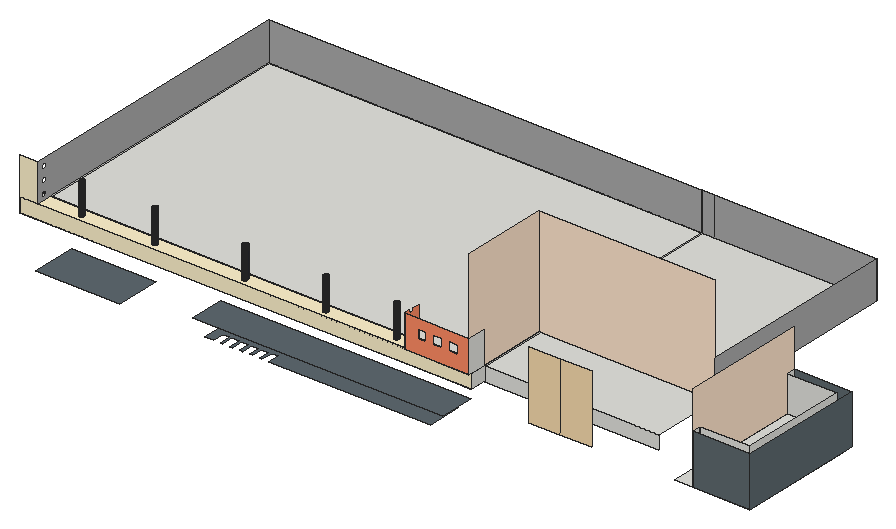
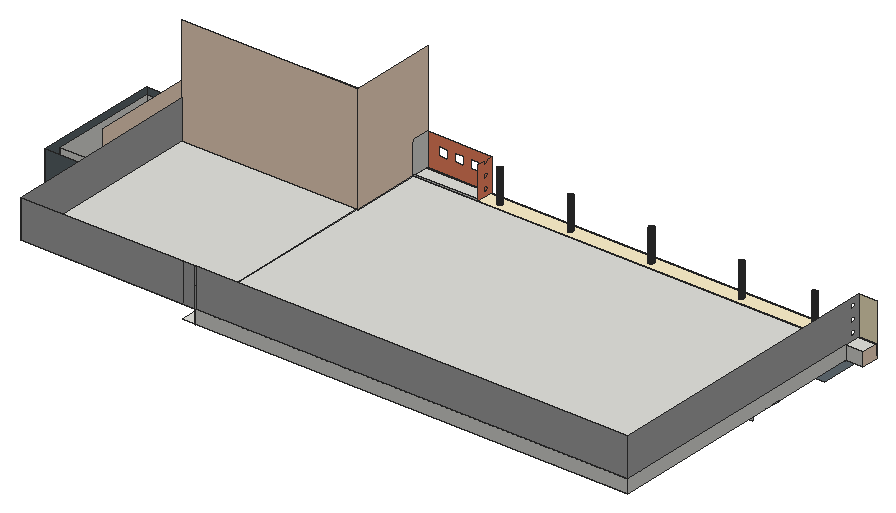
# SketchUp Ruby script. Lengths in inches.
U = 1.inch
M = Sketchup.active_model
def pt(a) = Geom::Point3d.new(a.map { |v| v * U })
def face(e, loops, mat)
  f = e.add_face(loops[0].map { |a| pt(a) })
  loops[1..].each { |l| e.add_face(l.map { |a| pt(a) }).erase! }
  f.material = f.back_material = mat if mat
  f
end
# faces: each face lists its corners as indices into pts; further lists are holes
def faces(e, pts, list, mat = nil) = list.each { |f| face(e, (f[0].is_a?(Array) ? f : [f]).map { |l| l.map { |i| pts[i] } }, mat) }
# xy, xz, yz: faces in a plane at the given z, y or x. An outline is a flat list of corners, or four numbers for a rectangle; further outlines are holes
def ring(l) = l.size == 4 ? [[l[0], l[1]], [l[2], l[1]], [l[2], l[3]], [l[0], l[3]]] : l.each_slice(2).to_a
def flat(e, list, mat, &to3) = list.each { |f| face(e, (f[0].is_a?(Array) ? f : [f]).map { |l| ring(l).map { |u, v| to3.(u, v) } }, mat) }
def xy(e, z, list, mat = nil) = flat(e, list, mat) { |x, y| [x, y, z] }
def xz(e, y, list, mat = nil) = flat(e, list, mat) { |x, z| [x, y, z] }
def yz(e, x, list, mat = nil) = flat(e, list, mat) { |y, z| [x, y, z] }
def lines(e, pts, list) = list.each { |a, b| e.add_line(pt(pts[a]), pt(pts[b])) }
# prism: a flat outline (further loops are holes) pulled along v
def prism(e, loops, v, mat = nil)
  f = face(e, loops, mat); d = Geom::Vector3d.new(v.map { |x| x * U })
  f.pushpull(f.normal.samedirection?(d) ? d.length : -d.length)
end
def box(e, o, s, mat = nil) = prism(e, [[o, [o[0] + s[0], o[1], o[2]], [o[0] + s[0], o[1] + s[1], o[2]], [o[0], o[1] + s[1], o[2]]]], [0, 0, s[2]], mat)
def at(x, y, z, deg = 0) = Geom::Transformation.translation(pt([x, y, z])) * Geom::Transformation.rotation(ORIGIN, Z_AXIS, deg.degrees)
def axes(o, x, y, z) = Geom::Transformation.new([*x, 0, *y, 0, *z, 0, *pt(o).to_a, 1])
def part(name) = M.definitions.add(name)
# library, detail: a bought-in or finely detailed component or shape, given as its bounding box
def library(name, o, s) = part(name).tap { |d| box(d.entities, o, s) }
def detail(e, o, s) = box(e.add_group.entities, o, s)
def put(e, d, t, mat = nil) = e.add_instance(d, t).tap { |i| i.material = mat if mat }
def group(e, t, mat = nil) = e.add_group.tap { |g| g.transformation = t; g.material = mat if mat }.entities
root = M.entities
M.materials.add("[Color B03]").color = [255, 140, 101]
M.materials.add("[Color C01]1").color = [255, 229, 204]
M.materials.add("[Color D01]").color = [255, 242, 204]
M.materials.add("[Color M03]").color = [170, 170, 170]
M.materials.add("[Formica Beige]1").color = [247, 219, 174]
M.materials.add("[Formica Laminate Dark]").color = [50, 53, 60]
M.materials.add("[Formica Speckled Grey]").color = [94, 105, 111]
xy(root,885.007,[[1665.331,219.809,1713.027,557.621],[1713.027,528.448,1866.152,557.621]])
xy(root,885.007,[[[1713.027,219.809,1713.027,240.489,1736.964,240.489,1736.964,274.614,1713.027,274.614,1713.027,528.448,1866.152,528.448,1866.152,219.809],[1750.402,240.489,1774.339,274.614],[1790.964,240.489,1814.902,274.614],[1823.339,240.489,1847.277,274.614]]],"[Formica Speckled Grey]")
xy(root,892.389,[[531.184,73.923,531.184,166.105,1131.08,166.105,1131.08,73.923,701.834,73.923,701.834,104.16,683.146,104.16,683.146,73.923,676.459,73.923,676.459,104.16,657.771,104.16,657.771,73.923,650.271,73.923,650.271,104.16,631.584,104.16,631.584,73.923,623.459,73.923,623.459,104.16,604.771,104.16,604.771,73.923,597.959,73.923,597.959,104.16,579.271,104.16,579.271,73.923,572.521,73.923,572.521,104.16,553.834,104.16,553.834,73.923]],"[Formica Speckled Grey]")
xy(root,911.081,[[100.986,47.542,326.111,166.105]],"[Formica Speckled Grey]")
xy(root,922.568,[[1713.027,243.888,1844.714,533.576]])
xy(root,925.697,[[497.875,73.923,1164.389,166.105]],"[Formica Speckled Grey]")
xy(root,980.3125,[[1198.268,166.042,1198.268,166.105,451.357,166.105,451.357,166.083,497.875,166.08],[1201.787,166.042,1232.713,890.389],[451.357,166.083,451.357,166.105,47.696,166.105],[1198.268,351.292,1201.787,388.542],[47.696,388.542,1201.412,388.542,1201.412,890.389,1198.268,890.389,1198.268,436.378,47.696,436.378]])
xy(root,980.9375,[[0,122.542,0,166.105,47.696,166.105,412.335,166.085,412.335,122.542],[412.335,122.542,412.335,166.085,451.311,166.083,451.311,122.542],[451.311,122.542,451.311,166.083,497.875,166.08,1159.05,166.044,1159.05,122.542],[1159.05,122.542,1159.05,166.044,1198.268,166.042,1198.268,122.542],[1198.268,122.542,1201.787,890.389],
  [1198.268,166.042,1159.05,166.044,1159.05,436.378,1198.268,436.378],[1159.05,166.044,497.875,166.08,451.311,166.083,451.311,436.378,1159.05,436.378],[451.311,166.083,412.335,166.085,412.335,436.378,451.311,436.378],[412.335,166.085,47.696,166.105,47.696,436.378,412.335,436.378],[47.696,436.378,412.335,890.389],
  [412.335,436.378,451.311,890.389],[451.311,436.378,1159.05,890.389],[1159.05,436.378,1198.268,890.389]])
xy(root,1016.9375,[[1025.893,119.173,1198.268,122.542],[0,122.542,47.696,166.105],[1198.268,122.542,1201.787,122.542,1201.787,890.389,47.696,890.389,47.696,166.105,1198.268,166.042],[1025.893,122.542,1198.268,166.042],[147.908,137.16,146.226,137.382,144.658,138.031,143.312,139.064,142.279,140.41,141.63,141.978,141.408,143.66,141.63,145.343,142.279,146.91,143.312,148.257,144.658,149.289,146.226,149.939,147.908,150.16,149.591,149.939,151.158,149.289,152.504,148.257,153.537,146.91,154.187,145.343,154.408,143.66,154.187,141.978,153.537,140.41,152.504,139.064,151.158,138.031,149.591,137.382],
  [341.783,137.16,340.101,137.382,338.533,138.031,337.187,139.064,336.154,140.41,335.505,141.978,335.283,143.66,335.505,145.343,336.154,146.91,337.187,148.257,338.533,149.289,340.101,149.939,341.783,150.16,343.466,149.939,345.033,149.289,346.379,148.257,347.412,146.91,348.062,145.343,348.283,143.66,348.062,141.978,347.412,140.41,346.379,139.064,345.033,138.031,343.466,137.382],[582.033,137.16,580.351,137.382,578.783,138.031,577.437,139.064,576.404,140.41,575.755,141.978,575.533,143.66,575.755,145.343,576.404,146.91,577.437,148.257,578.783,149.289,580.351,149.939,582.033,150.16,583.716,149.939,585.283,149.289,586.629,148.257,587.662,146.91,588.312,145.343,588.533,143.66,588.312,141.978,587.662,140.41,586.629,139.064,585.283,138.031,583.716,137.382],[797.721,137.16,796.038,137.382,794.471,138.031,793.125,139.064,792.092,140.41,791.442,141.978,791.221,143.66,791.442,145.343,792.092,146.91,793.125,148.257,794.471,149.289,796.038,149.939,797.721,150.16,799.403,149.939,800.971,149.289,802.317,148.257,803.35,146.91,803.999,145.343,804.221,143.66,803.999,141.978,803.35,140.41,802.317,139.064,800.971,138.031,799.403,137.382],[984.137,138.709,982.455,138.93,980.887,139.58,979.541,140.613,978.508,141.959,977.859,143.527,977.637,145.209,977.859,146.891,978.508,148.459,979.541,149.805,980.887,150.838,982.455,151.487,984.137,151.709,985.819,151.487,987.387,150.838,988.733,149.805,989.766,148.459,990.416,146.891,990.637,145.209,990.416,143.527,989.766,141.959,988.733,140.613,987.387,139.58,985.819,138.93],[1201.787,166.042,1665.331,351.292],
  [1201.787,351.292,1665.331,890.389]])
xy(root,1016.9375,[[[47.696,122.542,1025.893,122.542,1025.893,166.042,1198.268,166.042,47.696,166.105],[984.137,138.709,982.455,138.93,980.887,139.58,979.541,140.613,978.508,141.959,977.859,143.527,977.637,145.209,977.859,146.891,978.508,148.459,979.541,149.805,980.887,150.838,982.455,151.487,984.137,151.709,985.819,151.487,987.387,150.838,988.733,149.805,989.766,148.459,990.416,146.891,990.637,145.209,990.416,143.527,989.766,141.959,988.733,140.613,987.387,139.58,985.819,138.93],[341.783,137.16,340.101,137.382,338.533,138.031,337.187,139.064,336.154,140.41,335.505,141.978,335.283,143.66,335.505,145.343,336.154,146.91,337.187,148.257,338.533,149.289,340.101,149.939,341.783,150.16,343.466,149.939,345.033,149.289,346.379,148.257,347.412,146.91,348.062,145.343,348.283,143.66,348.062,141.978,347.412,140.41,346.379,139.064,345.033,138.031,343.466,137.382],[797.721,137.16,796.038,137.382,794.471,138.031,793.125,139.064,792.092,140.41,791.442,141.978,791.221,143.66,791.442,145.343,792.092,146.91,793.125,148.257,794.471,149.289,796.038,149.939,797.721,150.16,799.403,149.939,800.971,149.289,802.317,148.257,803.35,146.91,803.999,145.343,804.221,143.66,803.999,141.978,803.35,140.41,802.317,139.064,800.971,138.031,799.403,137.382],[582.033,137.16,580.351,137.382,578.783,138.031,577.437,139.064,576.404,140.41,575.755,141.978,575.533,143.66,575.755,145.343,576.404,146.91,577.437,148.257,578.783,149.289,580.351,149.939,582.033,150.16,583.716,149.939,585.283,149.289,586.629,148.257,587.662,146.91,588.312,145.343,588.533,143.66,588.312,141.978,587.662,140.41,586.629,139.064,585.283,138.031,583.716,137.382],[147.908,137.16,146.226,137.382,144.658,138.031,143.312,139.064,142.279,140.41,141.63,141.978,141.408,143.66,141.63,145.343,142.279,146.91,143.312,148.257,144.658,149.289,146.226,149.939,147.908,150.16,149.591,149.939,151.158,149.289,152.504,148.257,153.537,146.91,154.187,145.343,154.408,143.66,154.187,141.978,153.537,140.41,152.504,139.064,151.158,138.031,149.591,137.382]]],"[Color D01]")
xz(root,119.173,[[[1025.893,1016.9375,1198.268,1102.645],[1060.122,1053.817,1083.872,1077.567],[1102.122,1053.817,1125.872,1077.567],[1144.684,1053.817,1168.434,1077.567]]],"[Color B03]")
xz(root,119.173,[[1358.015,957.692,1440.68,1139.823],[1440.68,957.692,1523.345,1139.823]],"[Formica Beige]1")
xz(root,122.542,[[0,980.9375,1201.787,1016.9375],[0,1016.9375,47.696,1119.0625]],"[Color D01]")
xz(root,166.042,[[1201.787,980.3125,1665.331,1016.9375],[1025.893,1016.9375,1198.268,1021.906]])
xz(root,166.105,[[0,980.9375,47.696,1016.9375]])
xz(root,219.809,[[1713.027,885.007,1866.152,1017.818]],"[Formica Speckled Grey]")
xz(root,243.888,[[1713.027,922.568,1844.714,1017.818]])
xz(root,351.292,[[1198.268,980.3125,1198.268,1305.375,1665.331,1305.375,1665.331,1016.9375,1201.787,1016.9375,1201.787,980.3125]],"[Color C01]1")
xz(root,388.542,[[116.162,908.992,307.287,929.242]])
xz(root,436.378,[[47.696,980.3125,412.335,980.9375],[412.335,980.3125,451.311,980.9375],[451.311,980.3125,1159.05,980.9375],[1159.05,980.3125,1198.268,980.9375]])
xz(root,533.576,[[1713.027,922.568,1844.714,1017.818]])
xz(root,557.621,[[1713.027,885.007,1866.152,1017.818]],"[Formica Speckled Grey]")
xz(root,890.389,[[47.696,980.9375,1201.787,1016.9375]])
xz(root,890.389,[[47.696,1016.9375,1198.268,1119.0625],[1198.268,1016.9375,1201.787,1119.0625],[1201.787,1016.9375,1232.713,1119.0625],[1232.713,1016.9375,1665.331,1119.0625]],"[Color M03]")
yz(root,0,[[122.542,980.9375,166.105,1016.9375]],"[Color C01]1")
yz(root,47.696,[[388.542,980.3125,436.378,980.9375],[166.105,980.9375,890.389,1016.9375]])
yz(root,47.696,[[[122.542,1016.9375,890.389,1119.0625],[141.311,1027.741,139.531,1027.975,137.873,1028.662,136.449,1029.754,135.357,1031.178,134.67,1032.836,134.436,1034.616,134.67,1036.395,135.357,1038.053,136.449,1039.477,137.873,1040.57,139.531,1041.256,141.311,1041.491,143.09,1041.256,144.748,1040.57,146.172,1039.477,147.265,1038.053,147.952,1036.395,148.186,1034.616,147.952,1032.836,147.265,1031.178,146.172,1029.754,144.748,1028.662,143.09,1027.975],[141.311,1060.553,139.531,1060.787,137.873,1061.474,136.449,1062.567,135.357,1063.991,134.67,1065.649,134.436,1067.428,134.67,1069.208,135.357,1070.866,136.449,1072.29,137.873,1073.382,139.531,1074.069,141.311,1074.303,143.09,1074.069,144.748,1073.382,146.172,1072.29,147.265,1070.866,147.952,1069.208,148.186,1067.428,147.952,1065.649,147.265,1063.991,146.172,1062.567,144.748,1061.474,143.09,1060.787],[141.311,1093.991,139.531,1094.225,137.873,1094.912,136.449,1096.004,135.357,1097.428,134.67,1099.086,134.436,1100.866,134.67,1102.645,135.357,1104.303,136.449,1105.727,137.873,1106.82,139.531,1107.506,141.311,1107.741,143.09,1107.506,144.748,1106.82,146.172,1105.727,147.265,1104.303,147.952,1102.645,148.186,1100.866,147.952,1099.086,147.265,1097.428,146.172,1096.004,144.748,1094.912,143.09,1094.225]]],"[Color M03]")
yz(root,1025.893,[[[119.173,1016.9375,119.173,1102.645,134.67,1102.645,134.669,1102.638,134.436,1100.866,134.669,1099.094,134.67,1099.086,135.357,1097.428,136.449,1096.004,137.873,1094.912,139.531,1094.225,141.311,1093.991,143.09,1094.225,144.748,1094.912,146.172,1096.004,147.265,1097.428,147.952,1099.086,147.952,1099.094,148.186,1100.866,147.952,1102.638,147.952,1102.645,166.042,1102.645,166.042,1016.9375],[141.311,1060.553,143.09,1060.787,144.748,1061.474,146.172,1062.567,147.265,1063.991,147.952,1065.649,148.186,1067.428,147.952,1069.208,147.265,1070.866,146.172,1072.29,144.748,1073.382,143.09,1074.069,141.311,1074.303,139.531,1074.069,137.873,1073.382,136.449,1072.29,135.357,1070.866,134.67,1069.208,134.436,1067.428,134.67,1065.649,135.357,1063.991,136.449,1062.567,137.873,1061.474,139.531,1060.787],[141.311,1027.741,143.09,1027.975,144.748,1028.662,146.172,1029.754,147.265,1031.178,147.952,1032.836,148.186,1034.616,147.952,1036.395,147.265,1038.053,146.172,1039.477,144.748,1040.57,143.09,1041.256,141.311,1041.491,139.531,1041.256,137.873,1040.57,136.449,1039.477,135.357,1038.053,134.67,1036.395,134.436,1034.616,134.67,1032.836,135.357,1031.178,136.449,1029.754,137.873,1028.662,139.531,1027.975]]],"[Color B03]")
yz(root,1198.268,[[166.042,980.3125,351.292,980.9375],[436.378,980.3125,890.389,980.9375],[166.042,980.9375,351.292,1016.9375],[119.173,1016.9375,166.042,1102.645]])
yz(root,1198.268,[[166.042,1016.9375,166.042,1102.645,119.173,1102.645,119.173,1305.375,351.292,1305.375,351.292,1016.9375]],"[Color C01]1")
yz(root,1201.787,[[166.042,980.3125,351.292,980.9375],[122.542,980.9375,166.042,1016.9375],[166.042,980.9375,351.292,1016.9375],[351.292,980.9375,890.389,1016.9375]])
yz(root,1665.331,[[351.292,1016.9375,890.389,1119.0625]],"[Color M03]")
yz(root,1713.027,[[219.809,885.007,219.809,1017.818,243.888,1017.818,243.888,922.568,533.576,922.568,533.576,1017.818,557.621,1017.818,557.621,885.007]])
yz(root,1713.027,[[243.888,922.568,533.576,922.568,533.576,1017.818,557.621,1017.818,557.621,1119.0625,219.809,1119.0625,219.809,1017.818,243.888,1017.818]],"[Color C01]1")
yz(root,1844.714,[[243.888,922.568,533.576,1017.818]])
yz(root,1866.152,[[219.809,885.007,557.621,1017.818]],"[Formica Speckled Grey]")
p = [[1159.05,166.044,980.9375],[497.875,166.08,980.9375],[497.875,166.08,980.3125],[1198.268,166.042,980.3125],[1198.268,166.042,980.9375],[451.357,166.083,980.3125],
  [451.311,166.083,980.9375],[412.335,166.085,980.9375],[47.696,166.105,980.9375],[47.696,166.105,980.3125],[1198.268,166.042,1016.9375],[47.696,166.105,1016.9375],
  [146.226,137.382,1016.9375],[147.908,137.16,1016.9375],[147.908,137.16,1099.25],[146.226,137.382,1099.25],[149.591,137.382,1016.9375],[149.591,137.382,1099.25],
  [340.101,137.382,1016.9375],[341.783,137.16,1016.9375],[341.783,137.16,1104.303],[340.101,137.382,1104.303],[343.466,137.382,1016.9375],[343.466,137.382,1104.303],
  [580.351,137.382,1016.9375],[582.033,137.16,1016.9375],[582.033,137.16,1100.625],[580.351,137.382,1100.625],[583.716,137.382,1016.9375],[583.716,137.382,1100.625],
  [796.038,137.382,1016.9375],[797.721,137.16,1016.9375],[797.721,137.16,1101.75],[796.038,137.382,1101.75],[799.403,137.382,1016.9375],[799.403,137.382,1101.75],
  [144.658,138.031,1016.9375],[144.658,138.031,1099.25],[151.158,138.031,1016.9375],[151.158,138.031,1099.25],[338.533,138.031,1016.9375],[338.533,138.031,1104.303],
  [345.033,138.031,1016.9375],[345.033,138.031,1104.303],[578.783,138.031,1016.9375],[578.783,138.031,1100.625],[585.283,138.031,1016.9375],[585.283,138.031,1100.625],
  [794.471,138.031,1016.9375],[794.471,138.031,1101.75],[800.971,138.031,1016.9375],[800.971,138.031,1101.75],[143.312,139.064,1016.9375],[143.312,139.064,1099.25],
  [152.504,139.064,1016.9375],[152.504,139.064,1099.25],[337.187,139.064,1016.9375],[337.187,139.064,1104.303],[346.379,139.064,1016.9375],[346.379,139.064,1104.303],
  [577.437,139.064,1016.9375],[577.437,139.064,1100.625],[586.629,139.064,1016.9375],[586.629,139.064,1100.625],[793.125,139.064,1016.9375],[793.125,139.064,1101.75],
  [802.317,139.064,1016.9375],[802.317,139.064,1101.75],[982.455,138.93,1016.9375],[984.137,138.709,1016.9375],[984.137,138.709,1101.75],[982.455,138.93,1101.75],
  [985.819,138.93,1016.9375],[985.819,138.93,1101.75],[980.887,139.58,1016.9375],[980.887,139.58,1101.75],[987.387,139.58,1016.9375],[987.387,139.58,1101.75],
  [142.279,140.41,1016.9375],[142.279,140.41,1099.25],[153.537,140.41,1016.9375],[153.537,140.41,1099.25],[336.154,140.41,1016.9375],[336.154,140.41,1104.303],
  [347.412,140.41,1016.9375],[347.412,140.41,1104.303],[576.404,140.41,1016.9375],[576.404,140.41,1100.625],[587.662,140.41,1016.9375],[587.662,140.41,1100.625],
  [792.092,140.41,1016.9375],[792.092,140.41,1101.75],[803.35,140.41,1016.9375],[803.35,140.41,1101.75],[979.541,140.613,1016.9375],[979.541,140.613,1101.75],
  [988.733,140.613,1016.9375],[988.733,140.613,1101.75],[141.63,141.978,1016.9375],[141.63,141.978,1099.25],[154.187,141.978,1016.9375],[154.187,141.978,1099.25],
  [335.505,141.978,1016.9375],[335.505,141.978,1104.303],[348.062,141.978,1016.9375],[348.062,141.978,1104.303],[575.755,141.978,1016.9375],[575.755,141.978,1100.625],
  [588.312,141.978,1016.9375],[588.312,141.978,1100.625],[791.442,141.978,1016.9375],[791.442,141.978,1101.75],[803.999,141.978,1016.9375],[803.999,141.978,1101.75],
  [978.508,141.959,1016.9375],[978.508,141.959,1101.75],[989.766,141.959,1016.9375],[989.766,141.959,1101.75],[141.408,143.66,1016.9375],[141.408,143.66,1099.25],
  [154.408,143.66,1016.9375],[154.408,143.66,1099.25],[335.283,143.66,1016.9375],[335.283,143.66,1104.303],[348.283,143.66,1016.9375],[348.283,143.66,1104.303],
  [575.533,143.66,1016.9375],[575.533,143.66,1100.625],[588.533,143.66,1016.9375],[588.533,143.66,1100.625],[791.221,143.66,1016.9375],[791.221,143.66,1101.75],
  [804.221,143.66,1016.9375],[804.221,143.66,1101.75],[977.859,143.527,1016.9375],[977.859,143.527,1101.75],[990.416,143.527,1016.9375],[990.416,143.527,1101.75],
  [977.637,145.209,1016.9375],[977.637,145.209,1101.75],[990.637,145.209,1016.9375],[990.637,145.209,1101.75],[141.63,145.343,1016.9375],[141.63,145.343,1099.25],
  [154.187,145.343,1016.9375],[154.187,145.343,1099.25],[335.505,145.343,1016.9375],[335.505,145.343,1104.303],[348.062,145.343,1016.9375],[348.062,145.343,1104.303],
  [575.755,145.343,1016.9375],[575.755,145.343,1100.625],[588.312,145.343,1016.9375],[588.312,145.343,1100.625],[791.442,145.343,1016.9375],[791.442,145.343,1101.75],
  [803.999,145.343,1016.9375],[803.999,145.343,1101.75],[977.859,146.891,1016.9375],[977.859,146.891,1101.75],[990.416,146.891,1016.9375],[990.416,146.891,1101.75],
  [142.279,146.91,1016.9375],[142.279,146.91,1099.25],[153.537,146.91,1016.9375],[153.537,146.91,1099.25],[336.154,146.91,1016.9375],[336.154,146.91,1104.303],
  [347.412,146.91,1016.9375],[347.412,146.91,1104.303],[576.404,146.91,1016.9375],[576.404,146.91,1100.625],[587.662,146.91,1016.9375],[587.662,146.91,1100.625],
  [792.092,146.91,1016.9375],[792.092,146.91,1101.75],[803.35,146.91,1016.9375],[803.35,146.91,1101.75],[143.312,148.257,1016.9375],[143.312,148.257,1099.25],
  [152.504,148.257,1016.9375],[152.504,148.257,1099.25],[337.187,148.257,1016.9375],[336.426,147.265,1104.303],[337.187,148.257,1104.303],[346.379,148.257,1016.9375],
  [346.379,148.257,1104.303],[347.14,147.265,1104.303],[577.437,148.257,1016.9375],[577.437,148.257,1100.625],[586.629,148.257,1016.9375],[586.629,148.257,1100.625],
  [793.125,148.257,1016.9375],[793.125,148.257,1101.75],[802.317,148.257,1016.9375],[802.317,148.257,1101.75],[978.508,148.459,1016.9375],[978.508,148.459,1101.75],
  [989.766,148.459,1016.9375],[989.766,148.459,1101.75],[144.658,149.289,1016.9375],[144.658,149.289,1099.25],[151.158,149.289,1016.9375],[151.158,149.289,1099.25],
  [338.533,149.289,1016.9375],[338.533,149.289,1104.303],[345.033,149.289,1016.9375],[345.033,149.289,1104.303],[578.783,149.289,1016.9375],[578.783,149.289,1100.625],
  [585.283,149.289,1016.9375],[585.283,149.289,1100.625],[794.471,149.289,1016.9375],[794.471,149.289,1101.75],[800.971,149.289,1016.9375],[800.971,149.289,1101.75],
  [979.541,149.805,1016.9375],[979.541,149.805,1101.75],[988.733,149.805,1016.9375],[988.733,149.805,1101.75],[146.226,149.939,1016.9375],[146.226,149.939,1099.25],
  [149.591,149.939,1016.9375],[149.591,149.939,1099.25],[340.101,149.939,1016.9375],[340.101,149.939,1104.303],[343.466,149.939,1016.9375],[343.466,149.939,1104.303],
  [580.351,149.939,1016.9375],[580.351,149.939,1100.625],[583.716,149.939,1016.9375],[583.716,149.939,1100.625],[796.038,149.939,1016.9375],[796.038,149.939,1101.75],
  [799.403,149.939,1016.9375],[799.403,149.939,1101.75],[980.887,150.838,1016.9375],[980.887,150.838,1101.75],[987.387,150.838,1016.9375],[987.387,150.838,1101.75],
  [147.908,150.16,1016.9375],[147.908,150.16,1099.25],[341.783,150.16,1016.9375],[341.783,150.16,1104.303],[582.033,150.16,1016.9375],[582.033,150.16,1100.625],
  [797.721,150.16,1016.9375],[797.721,150.16,1101.75],[982.455,151.487,1016.9375],[982.455,151.487,1101.75],[985.819,151.487,1016.9375],[985.819,151.487,1101.75],
  [984.137,151.709,1016.9375],[984.137,151.709,1101.75]]
faces(root,p,[[0,1,2,3,4],[5,2,1,6,7,8,9],[10,11,8,7,6,1,0,4]])
faces(root,p,[[12,13,14,15],[13,16,17,14],[18,19,20,21],[19,22,23,20],[24,25,26,27],[25,28,29,26],[30,31,32,33],[31,34,35,32],
  [36,12,15,37],[16,38,39,17],[40,18,21,41],[22,42,43,23],[44,24,27,45],[28,46,47,29],[48,30,33,49],[34,50,51,35],
  [52,36,37,53],[38,54,55,39],[56,40,41,57],[42,58,59,43],[60,44,45,61],[46,62,63,47],[64,48,49,65],[50,66,67,51],
  [68,69,70,71],[69,72,73,70],[74,68,71,75],[72,76,77,73],[78,52,53,79],[54,80,81,55],[82,56,57,83],[58,84,85,59],
  [86,60,61,87],[62,88,89,63],[90,64,65,91],[66,92,93,67],[94,74,75,95],[76,96,97,77],[98,78,79,99],[80,100,101,81],
  [102,82,83,103],[84,104,105,85],[106,86,87,107],[88,108,109,89],[110,90,91,111],[92,112,113,93],[114,94,95,115],[96,116,117,97],
  [118,98,99,119],[100,120,121,101],[122,102,103,123],[104,124,125,105],[126,106,107,127],[108,128,129,109],[130,110,111,131],[112,132,133,113],
  [134,114,115,135],[116,136,137,117],[138,134,135,139],[136,140,141,137],[142,118,119,143],[120,144,145,121],[146,122,123,147],[124,148,149,125],
  [150,126,127,151],[128,152,153,129],[154,130,131,155],[132,156,157,133],[158,138,139,159],[140,160,161,141],[162,142,143,163],[144,164,165,145],
  [166,146,147,167],[148,168,169,149],[170,150,151,171],[152,172,173,153],[174,154,155,175],[156,176,177,157],[178,162,163,179],[164,180,181,165],
  [182,166,167,183,184],[168,185,186,187,169],[188,170,171,189],[172,190,191,173],[192,174,175,193],[176,194,195,177],[196,158,159,197],[160,198,199,161],
  [200,178,179,201],[180,202,203,181],[204,182,184,205],[185,206,207,186],[208,188,189,209],[190,210,211,191],[212,192,193,213],[194,214,215,195],
  [216,196,197,217],[198,218,219,199],[220,200,201,221],[202,222,223,203],[224,204,205,225],[206,226,227,207],[228,208,209,229],[210,230,231,211],
  [232,212,213,233],[214,234,235,215],[236,216,217,237],[218,238,239,219],[240,220,221,241],[222,240,241,223],[242,224,225,243],[226,242,243,227],
  [244,228,229,245],[230,244,245,231],[246,232,233,247],[234,246,247,235],[248,236,237,249],[238,250,251,239],[252,248,249,253],[250,252,253,251]],"[Formica Laminate Dark]")
